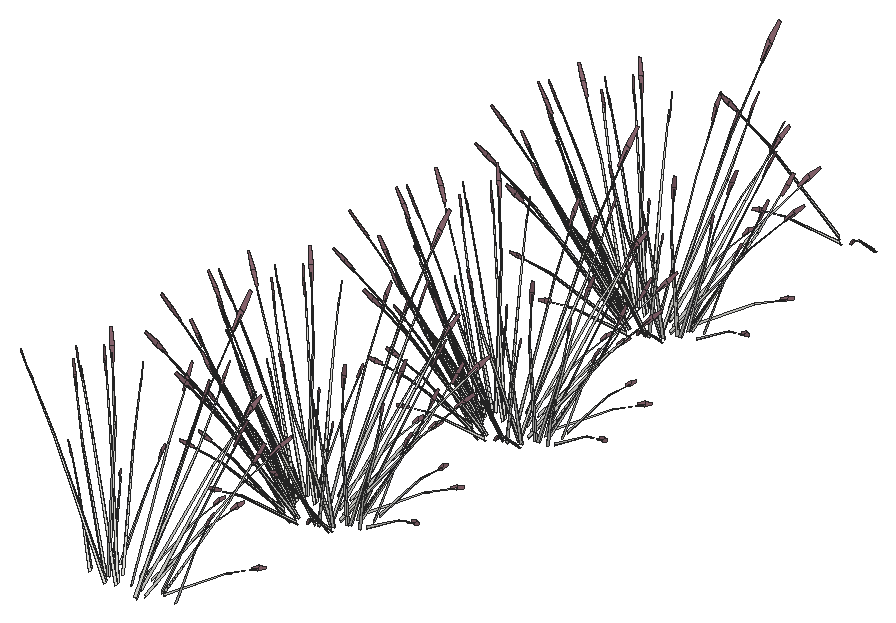
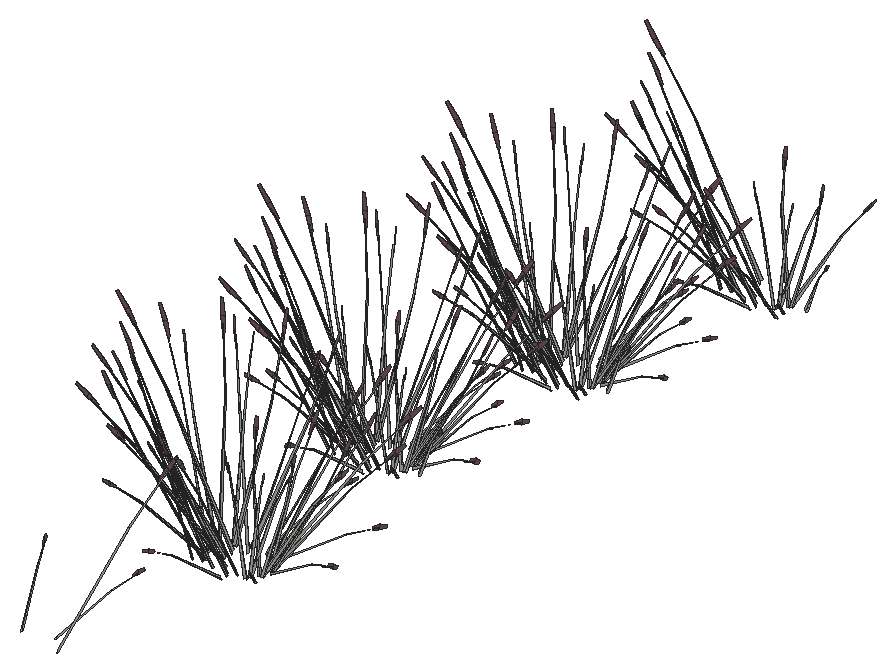
# SketchUp Ruby script. Lengths in inches.
U = 1.inch
M = Sketchup.active_model
def pt(a) = Geom::Point3d.new(a.map { |v| v * U })
def face(e, loops, mat)
  f = e.add_face(loops[0].map { |a| pt(a) })
  loops[1..].each { |l| e.add_face(l.map { |a| pt(a) }).erase! }
  f.material = f.back_material = mat if mat
  f
end
# faces: each face lists its corners as indices into pts; further lists are holes
def faces(e, pts, list, mat = nil) = list.each { |f| face(e, (f[0].is_a?(Array) ? f : [f]).map { |l| l.map { |i| pts[i] } }, mat) }
# xy, xz, yz: faces in a plane at the given z, y or x. An outline is a flat list of corners, or four numbers for a rectangle; further outlines are holes
def ring(l) = l.size == 4 ? [[l[0], l[1]], [l[2], l[1]], [l[2], l[3]], [l[0], l[3]]] : l.each_slice(2).to_a
def flat(e, list, mat, &to3) = list.each { |f| face(e, (f[0].is_a?(Array) ? f : [f]).map { |l| ring(l).map { |u, v| to3.(u, v) } }, mat) }
def xy(e, z, list, mat = nil) = flat(e, list, mat) { |x, y| [x, y, z] }
def xz(e, y, list, mat = nil) = flat(e, list, mat) { |x, z| [x, y, z] }
def yz(e, x, list, mat = nil) = flat(e, list, mat) { |y, z| [x, y, z] }
def lines(e, pts, list) = list.each { |a, b| e.add_line(pt(pts[a]), pt(pts[b])) }
# prism: a flat outline (further loops are holes) pulled along v
def prism(e, loops, v, mat = nil)
  f = face(e, loops, mat); d = Geom::Vector3d.new(v.map { |x| x * U })
  f.pushpull(f.normal.samedirection?(d) ? d.length : -d.length)
end
def box(e, o, s, mat = nil) = prism(e, [[o, [o[0] + s[0], o[1], o[2]], [o[0] + s[0], o[1] + s[1], o[2]], [o[0], o[1] + s[1], o[2]]]], [0, 0, s[2]], mat)
def at(x, y, z, deg = 0) = Geom::Transformation.translation(pt([x, y, z])) * Geom::Transformation.rotation(ORIGIN, Z_AXIS, deg.degrees)
def axes(o, x, y, z) = Geom::Transformation.new([*x, 0, *y, 0, *z, 0, *pt(o).to_a, 1])
def part(name) = M.definitions.add(name)
# library, detail: a bought-in or finely detailed component or shape, given as its bounding box
def library(name, o, s) = part(name).tap { |d| box(d.entities, o, s) }
def detail(e, o, s) = box(e.add_group.entities, o, s)
def put(e, d, t, mat = nil) = e.add_instance(d, t).tap { |i| i.material = mat if mat }
def group(e, t, mat = nil) = e.add_group.tap { |g| g.transformation = t; g.material = mat if mat }.entities
root = M.entities
M.materials.add("LightPink_Translucent").color = [144, 107, 117]
c1 = part("blade")
p = [[2.15,0.21,22],[0,0.17,0],[0.09,0.45,0],[2.18,0.31,22],[2.29,0.31,22],[0.38,0.45,0],
  [2.48,0.24,33],[2.49,0.24,33],[2.48,0.22,33]]
faces(c1.entities,p,[[0,1,2,3],[4,5,2,3],[6,3,4,7],[8,0,3,6]])
c2 = part("seeds")
p = [[0.3,-0.1,1.38],[-0.01,-0.03,1.59],[-0.01,-0.03,0.03],[0.14,-0.07,-0.07],[0.29,-0.03,3],[0.15,0.01,3.11]]
faces(c2.entities,p,[[0,1,2,3],[1,0,4,5]],"LightPink_Translucent")
c3 = part("blade with seeds")
put(c3.entities,c1,at(0,0,0))
put(c3.entities,c2,axes([2.4,0.25,30.99],[1.5799,-0.05474,1.17369],[-0.12525,1.92788,0.29478],[-0.07173,-0.02425,1.56792]))
put(root,c3,axes([41.28,395.99,45.93],[-0.23455,-0.87059,-0.03492],[1.10861,-0.20015,-0.15832],[0.23151,0.05519,0.52218]))
put(root,c3,axes([38.41,395.97,47.03],[0.06562,-1.05324,-0.1216],[1.2424,0.02879,-0.67495],[0.4785,0.07316,1.02557]))
put(root,c3,axes([39.49,395.34,46.72],[0.26289,-0.01751,1.74944],[0.72108,-0.8046,-0.27667],[0.46761,0.10621,0.14031]))
put(root,c3,axes([29.125,393.22,45.875],[0.42521,-0.21906,1.71376],[0.35798,1.01226,0.13857],[-0.66754,0.22878,0.73262]))
put(root,c3,axes([25.6,393.86,46.71],[0.1564,0.02778,1.77383],[0.48382,0.91506,-0.16761],[-0.32016,0.24017,0.31391]))
put(root,c3,axes([39.2,395.89,46.53],[0.69728,0.64842,-0.35414],[-0.79619,0.61382,0.4572],[0.40453,0.09339,0.87481]))
put(root,c3,axes([28.84,394.73,46.53],[-1.06674,0.14801,-0.35414],[-0.28168,-0.84611,0.4572],[-0.30569,0.22726,0.87481]))
put(root,c3,axes([36.7,394.23,45.875],[-0.45521,-0.17844,1.71376],[0.94204,-0.74856,0.13857],[0.58713,0.33769,0.73262]))
put(root,c3,axes([36.79,391.88,46.47],[-1.05895,-0.53811,1.38283],[1.11816,-0.83781,0.59665],[0.34166,0.5049,1.33663]))
put(root,c3,axes([29.15,394.15,47.03],[1.1336,0.57106,-0.1216],[-0.65308,0.827,-0.67495],[-0.32027,0.28747,1.02557]))
put(root,c3,axes([35.96,397.11,47.03],[0.73026,-0.88648,-0.1216],[1.05755,0.51071,-0.67495],[0.36761,0.25045,1.02557]))
put(root,c3,axes([30.68,393.9,45.875],[0.30609,-0.31822,1.71376],[0.77286,0.85893,0.13857],[-0.53009,0.39116,0.73262]))
put(root,c3,axes([35.01,397.85,46.71],[0.00363,-0.12539,1.77383],[1.0502,-0.55319,-0.16761],[0.36479,0.19745,0.31391]))
put(root,c3,axes([30.45,394.68,45.875],[0.22818,-0.35597,1.71376],[0.95725,0.73667,0.13857],[-0.43183,0.45914,0.73262]))
put(root,c3,axes([30.71,396.69,46.53],[-0.82919,0.54528,-0.35414],[-0.78493,-0.62262,0.4572],[-0.11943,0.31634,0.87481]))
put(root,c3,axes([27.86,396.53,46.72],[-0.03046,0.20495,1.74944],[0.86449,0.71297,-0.27667],[-0.22632,0.33716,0.14031]))
put(root,c3,axes([33.11,397.15,47.03],[1.19922,-0.48218,-0.1216],[0.58932,0.85579,-0.67495],[0.15822,0.36063,1.02557]))
put(root,c3,axes([34.82,395.27,45.875],[-0.28013,-0.33252,1.71376],[1.29445,-0.27994,0.13857],[0.29256,0.52202,0.73262]))
put(root,c3,axes([33.59,397.65,46.53],[-0.36946,0.79643,-0.35414],[-1.07787,-0.23229,0.4572],[0.09883,0.32066,0.87481]))
put(root,c3,axes([27.76,398.63,46.71],[0.13903,-0.06253,1.77383],[1.14912,0.41591,-0.16761],[-0.027,0.34629,0.31391]))
put(root,c3,axes([32.54,395.44,45.875],[-0.02999,-0.3975,1.71376],[1.30002,0.26369,0.13857],[-0.08041,0.56647,0.73262]))
put(root,c3,axes([32.83,399.06,46.72],[0.15534,0.16677,1.74944],[1.25362,0.06552,-0.27667],[0.12606,0.3678,0.14031]))
put(root,c3,axes([39.9,428.45,45.875],[0.28013,0.33252,1.71376],[-1.29445,0.27994,0.13857],[-0.29256,-0.52202,0.73262]))
put(root,c3,axes([42.04,426.25,46.72],[-0.18744,-0.14521,1.74944],[-1.25089,0.09206,-0.27667],[-0.19964,-0.34731,0.14031]))
put(root,c3,axes([47.66,428.03,46.72],[-0.01183,-0.20612,1.74944],[-0.99913,-0.59572,-0.27667],[0.15447,-0.36112,0.14031]))
put(root,c3,axes([43.46,427.98,46.53],[0.36946,-0.79643,-0.35414],[1.07787,0.23229,0.4572],[-0.09883,-0.32066,0.87481]))
put(root,c3,axes([44.28,429.04,45.875],[-0.22818,0.35597,1.71376],[-0.95725,-0.73667,0.13857],[0.43183,-0.45914,0.73262]))
put(root,c3,axes([47.39,427.29,46.71],[-0.12446,0.07911,1.77383],[-1.21937,-0.26689,-0.16761],[-0.04414,-0.34521,0.31391]))
put(root,c3,axes([40.76,425.77,46.71],[-0.02286,0.12414,1.77383],[-1.12758,0.45052,-0.16761],[-0.33182,-0.23029,0.31391]))
put(root,c3,axes([43.94,428.49,47.03],[-1.19922,0.48218,-0.1216],[-0.58932,-0.85579,-0.67495],[-0.15822,-0.36063,1.02557]))
put(root,c3,axes([46.43,429.57,47.03],[-1.34686,-0.05131,-0.1216],[0.03681,-0.97156,-0.67495],[0.09356,-0.37418,1.02557]))
put(root,c3,axes([46.34,428.95,46.53],[0.82919,-0.54528,-0.35414],[0.78493,0.62262,0.4572],[0.11943,-0.31634,0.87481]))
put(root,c3,axes([40.35,428.28,46.53],[-0.18927,-0.83419,-0.35414],[1.08199,-0.22027,0.4572],[-0.29062,-0.23905,0.87481]))
put(root,c3,axes([38.03,429.49,45.875],[0.45521,0.17844,1.71376],[-0.94204,0.74856,0.13857],[-0.58713,-0.33769,0.73262]))
put(root,c3,axes([37.9375,427.85,46.72],[-0.26368,-0.00731,1.74944],[-0.83946,0.73103,-0.27667],[-0.44791,-0.14937,0.14031]))
put(root,c3,axes([47.9,431.48,47.03],[-1.1336,-0.57106,-0.1216],[0.65308,-0.827,-0.67495],[0.32027,-0.28747,1.02557]))
put(root,c3,axes([50.69,431.24,46.71],[-0.16006,-0.00787,1.77383],[-0.66468,-0.8428,-0.16761],[0.26693,-0.27711,0.31391]))
put(root,c3,axes([48.22,430.91,46.53],[1.06674,-0.14801,-0.35414],[0.28168,0.84611,0.4572],[0.30569,-0.22726,0.87481]))
put(root,c3,axes([37.85,429.74,46.53],[-0.69728,-0.64842,-0.35414],[0.79619,-0.61382,0.4572],[-0.40453,-0.09339,0.87481]))
put(root,c3,axes([51.29,432.24,46.72],[0.17006,-0.15775,1.74944],[-0.21766,-0.96766,-0.27667],[0.42669,-0.18347,0.14031]))
put(root,c3,axes([36.92,428.47,46.71],[0.09085,0.10335,1.77383],[-0.43798,0.92907,-0.16761],[-0.44357,0.00672,0.31391]))
put(root,c3,axes([38.65,429.67,47.03],[-0.06562,1.05324,-0.1216],[-1.2424,-0.02879,-0.67495],[-0.4785,-0.07316,1.02557]))
put(root,c3,axes([47.94,433.71,47.03],[-0.6166,-0.93779,-0.1216],[1.09436,-0.46085,-0.67495],[0.46117,-0.12373,1.02557]))
put(root,c3,axes([37.07,431.12,45.875],[0.50831,-0.02346,1.71376],[-0.33721,1.01661,0.13857],[-0.72439,-0.06288,0.73262]))
put(root,c3,axes([48.59,433.34,46.53],[1.01846,0.28891,-0.35414],[-0.29705,0.84289,0.4572],[0.41005,-0.07729,0.87481]))
put(root,c3,axes([36.62,431.99,46.53],[-1.01846,-0.28891,-0.35414],[0.29705,-0.84289,0.4572],[-0.41005,0.07729,0.87481]))
put(root,c3,axes([45.8125,432.29,45.875],[-0.50831,0.02346,1.71376],[0.33721,-1.01661,0.13857],[0.72439,0.06288,0.73262]))
put(root,c3,axes([50.4,436.5,46.71],[-0.11081,-0.09067,1.77383],[0.2424,-0.97188,-0.16761],[0.43649,-0.06209,0.31391]))
put(root,c3,axes([35.98,432.55,46.72],[-0.20012,0.13446,1.74944],[0.01702,0.98243,-0.27667],[-0.45871,0.12776,0.14031]))
put(root,c3,axes([37.26,431.62,47.03],[0.6166,0.93779,-0.1216],[-1.09436,0.46085,-0.67495],[-0.46117,0.12373,1.02557]))
put(root,c3,axes([49.43,435.6875,45.93],[-0.23455,-0.87059,-0.03492],[1.10861,-0.20015,-0.15832],[0.23151,0.05519,0.52218]))
put(root,c3,axes([46.56,435.66,47.03],[0.06562,-1.05324,-0.1216],[1.2424,0.02879,-0.67495],[0.4785,0.07316,1.02557]))
put(root,c3,axes([47.64,435.03,46.72],[0.26289,-0.01751,1.74944],[0.72108,-0.8046,-0.27667],[0.46761,0.10621,0.14031]))
put(root,c3,axes([37.28,432.91,45.875],[0.42521,-0.21906,1.71376],[0.35798,1.01226,0.13857],[-0.66754,0.22878,0.73262]))
put(root,c3,axes([33.75,433.55,46.71],[0.1564,0.02778,1.77383],[0.48382,0.91506,-0.16761],[-0.32016,0.24017,0.31391]))
put(root,c3,axes([47.36,435.59,46.53],[0.69728,0.64842,-0.35414],[-0.79619,0.61382,0.4572],[0.40453,0.09339,0.87481]))
put(root,c3,axes([36.99,434.42,46.53],[-1.06674,0.14801,-0.35414],[-0.28168,-0.84611,0.4572],[-0.30569,0.22726,0.87481]))
put(root,c3,axes([44.85,433.92,45.875],[-0.45521,-0.17844,1.71376],[0.94204,-0.74856,0.13857],[0.58713,0.33769,0.73262]))
put(root,c3,axes([44.94,431.58,46.47],[-1.05895,-0.53811,1.38283],[1.11816,-0.83781,0.59665],[0.34166,0.5049,1.33663]))
put(root,c3,axes([37.31,433.85,47.03],[1.1336,0.57106,-0.1216],[-0.65308,0.827,-0.67495],[-0.32027,0.28747,1.02557]))
put(root,c3,axes([44.11,436.81,47.03],[0.73026,-0.88648,-0.1216],[1.05755,0.51071,-0.67495],[0.36761,0.25045,1.02557]))
put(root,c3,axes([38.83,433.59,45.875],[0.30609,-0.31822,1.71376],[0.77286,0.85893,0.13857],[-0.53009,0.39116,0.73262]))
put(root,c3,axes([43.16,437.54,46.71],[0.00363,-0.12539,1.77383],[1.0502,-0.55319,-0.16761],[0.36479,0.19745,0.31391]))
put(root,c3,axes([38.6,434.375,45.875],[0.22818,-0.35597,1.71376],[0.95725,0.73667,0.13857],[-0.43183,0.45914,0.73262]))
put(root,c3,axes([38.87,436.38,46.53],[-0.82919,0.54528,-0.35414],[-0.78493,-0.62262,0.4572],[-0.11943,0.31634,0.87481]))
put(root,c3,axes([36.01,436.22,46.72],[-0.03046,0.20495,1.74944],[0.86449,0.71297,-0.27667],[-0.22632,0.33716,0.14031]))
put(root,c3,axes([41.26,436.84,47.03],[1.19922,-0.48218,-0.1216],[0.58932,0.85579,-0.67495],[0.15822,0.36063,1.02557]))
put(root,c3,axes([42.98,434.96,45.875],[-0.28013,-0.33252,1.71376],[1.29445,-0.27994,0.13857],[0.29256,0.52202,0.73262]))
put(root,c3,axes([41.74,437.35,46.53],[-0.36946,0.79643,-0.35414],[-1.07787,-0.23229,0.4572],[0.09883,0.32066,0.87481]))
put(root,c3,axes([35.91,438.32,46.71],[0.13903,-0.06253,1.77383],[1.14912,0.41591,-0.16761],[-0.027,0.34629,0.31391]))
put(root,c3,axes([40.69,435.13,45.875],[-0.02999,-0.3975,1.71376],[1.30002,0.26369,0.13857],[-0.08041,0.56647,0.73262]))
put(root,c3,axes([40.98,438.76,46.72],[0.15534,0.16677,1.74944],[1.25362,0.06552,-0.27667],[0.12606,0.3678,0.14031]))
put(root,c3,axes([46.26,467.72,45.875],[0.28013,0.33252,1.71376],[-1.29445,0.27994,0.13857],[-0.29256,-0.52202,0.73262]))
put(root,c3,axes([48.39,465.51,46.72],[-0.18744,-0.14521,1.74944],[-1.25089,0.09206,-0.27667],[-0.19964,-0.34731,0.14031]))
put(root,c3,axes([54.01,467.29,46.72],[-0.01183,-0.20612,1.74944],[-0.99913,-0.59572,-0.27667],[0.15447,-0.36112,0.14031]))
put(root,c3,axes([49.82,467.25,46.53],[0.36946,-0.79643,-0.35414],[1.07787,0.23229,0.4572],[-0.09883,-0.32066,0.87481]))
put(root,c3,axes([50.63,468.3,45.875],[-0.22818,0.35597,1.71376],[-0.95725,-0.73667,0.13857],[0.43183,-0.45914,0.73262]))
put(root,c3,axes([47.11,465.04,46.71],[-0.02286,0.12414,1.77383],[-1.12758,0.45052,-0.16761],[-0.33182,-0.23029,0.31391]))
put(root,c3,axes([50.3,467.75,47.03],[-1.19922,0.48218,-0.1216],[-0.58932,-0.85579,-0.67495],[-0.15822,-0.36063,1.02557]))
put(root,c3,axes([52.79,468.84,47.03],[-1.34686,-0.05131,-0.1216],[0.03681,-0.97156,-0.67495],[0.09356,-0.37418,1.02557]))
put(root,c3,axes([52.69,468.21,46.53],[0.82919,-0.54528,-0.35414],[0.78493,0.62262,0.4572],[0.11943,-0.31634,0.87481]))
put(root,c3,axes([46.71,467.54,46.53],[-0.18927,-0.83419,-0.35414],[1.08199,-0.22027,0.4572],[-0.29062,-0.23905,0.87481]))
put(root,c3,axes([44.38,468.75,45.875],[0.45521,0.17844,1.71376],[-0.94204,0.74856,0.13857],[-0.58713,-0.33769,0.73262]))
put(root,c3,axes([44.29,467.11,46.72],[-0.26368,-0.00731,1.74944],[-0.83946,0.73103,-0.27667],[-0.44791,-0.14937,0.14031]))
put(root,c3,axes([54.25,470.75,47.03],[-1.1336,-0.57106,-0.1216],[0.65308,-0.827,-0.67495],[0.32027,-0.28747,1.02557]))
put(root,c3,axes([57.05,470.5,46.71],[-0.16006,-0.00787,1.77383],[-0.66468,-0.8428,-0.16761],[0.26693,-0.27711,0.31391]))
put(root,c3,axes([54.57,470.17,46.53],[1.06674,-0.14801,-0.35414],[0.28168,0.84611,0.4572],[0.30569,-0.22726,0.87481]))
put(root,c3,axes([44.2,469.01,46.53],[-0.69728,-0.64842,-0.35414],[0.79619,-0.61382,0.4572],[-0.40453,-0.09339,0.87481]))
put(root,c3,axes([57.65,471.51,46.72],[0.17006,-0.15775,1.74944],[-0.21766,-0.96766,-0.27667],[0.42669,-0.18347,0.14031]))
put(root,c3,axes([43.28,467.73,46.71],[0.09085,0.10335,1.77383],[-0.43798,0.92907,-0.16761],[-0.44357,0.00672,0.31391]))
put(root,c3,axes([45,468.93,47.03],[-0.06562,1.05324,-0.1216],[-1.2424,-0.02879,-0.67495],[-0.4785,-0.07316,1.02557]))
put(root,c3,axes([54.3,472.98,47.03],[-0.6166,-0.93779,-0.1216],[1.09436,-0.46085,-0.67495],[0.46117,-0.12373,1.02557]))
put(root,c3,axes([43.42,470.39,45.875],[0.50831,-0.02346,1.71376],[-0.33721,1.01661,0.13857],[-0.72439,-0.06288,0.73262]))
put(root,c3,axes([54.94,472.6,46.53],[1.01846,0.28891,-0.35414],[-0.29705,0.84289,0.4572],[0.41005,-0.07729,0.87481]))
put(root,c3,axes([42.97,471.26,46.53],[-1.01846,-0.28891,-0.35414],[0.29705,-0.84289,0.4572],[-0.41005,0.07729,0.87481]))
put(root,c3,axes([52.17,471.56,45.875],[-0.50831,0.02346,1.71376],[0.33721,-1.01661,0.13857],[0.72439,0.06288,0.73262]))
put(root,c3,axes([56.75,475.76,46.71],[-0.11081,-0.09067,1.77383],[0.2424,-0.97188,-0.16761],[0.43649,-0.06209,0.31391]))
put(root,c3,axes([42.33,471.82,46.72],[-0.20012,0.13446,1.74944],[0.01702,0.98243,-0.27667],[-0.45871,0.12776,0.14031]))
put(root,c3,axes([43.62,470.88,47.03],[0.6166,0.93779,-0.1216],[-1.09436,0.46085,-0.67495],[-0.46117,0.12373,1.02557]))
put(root,c3,axes([55.79,474.95,45.93],[-0.23455,-0.87059,-0.03492],[1.10861,-0.20015,-0.15832],[0.23151,0.05519,0.52218]))
put(root,c3,axes([52.92,474.93,47.03],[0.06562,-1.05324,-0.1216],[1.2424,0.02879,-0.67495],[0.4785,0.07316,1.02557]))
put(root,c3,axes([54,474.29,46.72],[0.26289,-0.01751,1.74944],[0.72108,-0.8046,-0.27667],[0.46761,0.10621,0.14031]))
put(root,c3,axes([43.63,472.17,45.875],[0.42521,-0.21906,1.71376],[0.35798,1.01226,0.13857],[-0.66754,0.22878,0.73262]))
put(root,c3,axes([40.11,472.8125,46.71],[0.1564,0.02778,1.77383],[0.48382,0.91506,-0.16761],[-0.32016,0.24017,0.31391]))
put(root,c3,axes([53.71,474.85,46.53],[0.69728,0.64842,-0.35414],[-0.79619,0.61382,0.4572],[0.40453,0.09339,0.87481]))
put(root,c3,axes([43.35,473.6875,46.53],[-1.06674,0.14801,-0.35414],[-0.28168,-0.84611,0.4572],[-0.30569,0.22726,0.87481]))
put(root,c3,axes([51.21,473.19,45.875],[-0.45521,-0.17844,1.71376],[0.94204,-0.74856,0.13857],[0.58713,0.33769,0.73262]))
put(root,c3,axes([51.3,470.84,46.47],[-1.05895,-0.53811,1.38283],[1.11816,-0.83781,0.59665],[0.34166,0.5049,1.33663]))
put(root,c3,axes([43.66,473.11,47.03],[1.1336,0.57106,-0.1216],[-0.65308,0.827,-0.67495],[-0.32027,0.28747,1.02557]))
put(root,c3,axes([50.47,476.07,47.03],[0.73026,-0.88648,-0.1216],[1.05755,0.51071,-0.67495],[0.36761,0.25045,1.02557]))
put(root,c3,axes([45.1875,472.86,45.875],[0.30609,-0.31822,1.71376],[0.77286,0.85893,0.13857],[-0.53009,0.39116,0.73262]))
put(root,c3,axes([49.51,476.81,46.71],[0.00363,-0.12539,1.77383],[1.0502,-0.55319,-0.16761],[0.36479,0.19745,0.31391]))
put(root,c3,axes([44.96,473.64,45.875],[0.22818,-0.35597,1.71376],[0.95725,0.73667,0.13857],[-0.43183,0.45914,0.73262]))
put(root,c3,axes([45.22,475.65,46.53],[-0.82919,0.54528,-0.35414],[-0.78493,-0.62262,0.4572],[-0.11943,0.31634,0.87481]))
put(root,c3,axes([42.36,475.49,46.72],[-0.03046,0.20495,1.74944],[0.86449,0.71297,-0.27667],[-0.22632,0.33716,0.14031]))
put(root,c3,axes([47.62,476.11,47.03],[1.19922,-0.48218,-0.1216],[0.58932,0.85579,-0.67495],[0.15822,0.36063,1.02557]))
put(root,c3,axes([49.33,474.23,45.875],[-0.28013,-0.33252,1.71376],[1.29445,-0.27994,0.13857],[0.29256,0.52202,0.73262]))
put(root,c3,axes([48.1,476.61,46.53],[-0.36946,0.79643,-0.35414],[-1.07787,-0.23229,0.4572],[0.09883,0.32066,0.87481]))
put(root,c3,axes([47.05,474.39,45.875],[-0.02999,-0.3975,1.71376],[1.30002,0.26369,0.13857],[-0.08041,0.56647,0.73262]))
put(root,c3,axes([47.34,478.02,46.72],[0.15534,0.16677,1.74944],[1.25362,0.06552,-0.27667],[0.12606,0.3678,0.14031]))
put(root,c3,axes([42.64,507.97,45.875],[0.28013,0.33252,1.71376],[-1.29445,0.27994,0.13857],[-0.29256,-0.52202,0.73262]))
put(root,c3,axes([44.78,505.77,46.72],[-0.18744,-0.14521,1.74944],[-1.25089,0.09206,-0.27667],[-0.19964,-0.34731,0.14031]))
put(root,c3,axes([50.4,507.55,46.72],[-0.01183,-0.20612,1.74944],[-0.99913,-0.59572,-0.27667],[0.15447,-0.36112,0.14031]))
put(root,c3,axes([46.2,507.51,46.53],[0.36946,-0.79643,-0.35414],[1.07787,0.23229,0.4572],[-0.09883,-0.32066,0.87481]))
put(root,c3,axes([47.02,508.5625,45.875],[-0.22818,0.35597,1.71376],[-0.95725,-0.73667,0.13857],[0.43183,-0.45914,0.73262]))
put(root,c3,axes([46.68,508.01,47.03],[-1.19922,0.48218,-0.1216],[-0.58932,-0.85579,-0.67495],[-0.15822,-0.36063,1.02557]))
put(root,c3,axes([49.17,509.09,47.03],[-1.34686,-0.05131,-0.1216],[0.03681,-0.97156,-0.67495],[0.09356,-0.37418,1.02557]))
put(root,c3,axes([49.08,508.47,46.53],[0.82919,-0.54528,-0.35414],[0.78493,0.62262,0.4572],[0.11943,-0.31634,0.87481]))
put(root,c3,axes([43.09,507.8,46.53],[-0.18927,-0.83419,-0.35414],[1.08199,-0.22027,0.4572],[-0.29062,-0.23905,0.87481]))
put(root,c3,axes([40.77,509.01,45.875],[0.45521,0.17844,1.71376],[-0.94204,0.74856,0.13857],[-0.58713,-0.33769,0.73262]))
put(root,c3,axes([40.68,507.37,46.72],[-0.26368,-0.00731,1.74944],[-0.83946,0.73103,-0.27667],[-0.44791,-0.14937,0.14031]))
put(root,c3,axes([50.64,511.01,47.03],[-1.1336,-0.57106,-0.1216],[0.65308,-0.827,-0.67495],[0.32027,-0.28747,1.02557]))
put(root,c3,axes([50.96,510.43,46.53],[1.06674,-0.14801,-0.35414],[0.28168,0.84611,0.4572],[0.30569,-0.22726,0.87481]))
put(root,c3,axes([40.59,509.27,46.53],[-0.69728,-0.64842,-0.35414],[0.79619,-0.61382,0.4572],[-0.40453,-0.09339,0.87481]))
put(root,c3,axes([54.03,511.77,46.72],[0.17006,-0.15775,1.74944],[-0.21766,-0.96766,-0.27667],[0.42669,-0.18347,0.14031]))
put(root,c3,axes([41.39,509.19,47.03],[-0.06562,1.05324,-0.1216],[-1.2424,-0.02879,-0.67495],[-0.4785,-0.07316,1.02557]))
put(root,c3,axes([50.69,513.24,47.03],[-0.6166,-0.93779,-0.1216],[1.09436,-0.46085,-0.67495],[0.46117,-0.12373,1.02557]))
put(root,c3,axes([39.81,510.64,45.875],[0.50831,-0.02346,1.71376],[-0.33721,1.01661,0.13857],[-0.72439,-0.06288,0.73262]))
put(root,c3,axes([51.33,512.86,46.53],[1.01846,0.28891,-0.35414],[-0.29705,0.84289,0.4572],[0.41005,-0.07729,0.87481]))
put(root,c3,axes([39.36,511.52,46.53],[-1.01846,-0.28891,-0.35414],[0.29705,-0.84289,0.4572],[-0.41005,0.07729,0.87481]))
put(root,c3,axes([48.55,511.82,45.875],[-0.50831,0.02346,1.71376],[0.33721,-1.01661,0.13857],[0.72439,0.06288,0.73262]))
put(root,c3,axes([38.72,512.08,46.72],[-0.20012,0.13446,1.74944],[0.01702,0.98243,-0.27667],[-0.45871,0.12776,0.14031]))
put(root,c3,axes([40,511.14,47.03],[0.6166,0.93779,-0.1216],[-1.09436,0.46085,-0.67495],[-0.46117,0.12373,1.02557]))
put(root,c3,axes([52.17,515.21,45.93],[-0.23455,-0.87059,-0.03492],[1.10861,-0.20015,-0.15832],[0.23151,0.05519,0.52218]))
put(root,c3,axes([49.3,515.18,47.03],[0.06562,-1.05324,-0.1216],[1.2424,0.02879,-0.67495],[0.4785,0.07316,1.02557]))
put(root,c3,axes([50.38,514.55,46.72],[0.26289,-0.01751,1.74944],[0.72108,-0.8046,-0.27667],[0.46761,0.10621,0.14031]))
put(root,c3,axes([40.02,512.43,45.875],[0.42521,-0.21906,1.71376],[0.35798,1.01226,0.13857],[-0.66754,0.22878,0.73262]))
put(root,c3,axes([50.1,515.11,46.53],[0.69728,0.64842,-0.35414],[-0.79619,0.61382,0.4572],[0.40453,0.09339,0.87481]))
put(root,c3,axes([39.73,513.95,46.53],[-1.06674,0.14801,-0.35414],[-0.28168,-0.84611,0.4572],[-0.30569,0.22726,0.87481]))
put(root,c3,axes([47.59,513.45,45.875],[-0.45521,-0.17844,1.71376],[0.94204,-0.74856,0.13857],[0.58713,0.33769,0.73262]))
put(root,c3,axes([47.68,511.1,46.47],[-1.05895,-0.53811,1.38283],[1.11816,-0.83781,0.59665],[0.34166,0.5049,1.33663]))
put(root,c3,axes([40.05,513.37,47.03],[1.1336,0.57106,-0.1216],[-0.65308,0.827,-0.67495],[-0.32027,0.28747,1.02557]))
put(root,c3,axes([46.85,516.33,47.03],[0.73026,-0.88648,-0.1216],[1.05755,0.51071,-0.67495],[0.36761,0.25045,1.02557]))
put(root,c3,axes([41.57,513.11,45.875],[0.30609,-0.31822,1.71376],[0.77286,0.85893,0.13857],[-0.53009,0.39116,0.73262]))
put(root,c3,axes([41.34,513.9,45.875],[0.22818,-0.35597,1.71376],[0.95725,0.73667,0.13857],[-0.43183,0.45914,0.73262]))
put(root,c3,axes([41.61,515.91,46.53],[-0.82919,0.54528,-0.35414],[-0.78493,-0.62262,0.4572],[-0.11943,0.31634,0.87481]))
put(root,c3,axes([38.75,515.75,46.72],[-0.03046,0.20495,1.74944],[0.86449,0.71297,-0.27667],[-0.22632,0.33716,0.14031]))
put(root,c3,axes([44,516.37,47.03],[1.19922,-0.48218,-0.1216],[0.58932,0.85579,-0.67495],[0.15822,0.36063,1.02557]))
put(root,c3,axes([45.72,514.49,45.875],[-0.28013,-0.33252,1.71376],[1.29445,-0.27994,0.13857],[0.29256,0.52202,0.73262]))
put(root,c3,axes([44.49,516.87,46.53],[-0.36946,0.79643,-0.35414],[-1.07787,-0.23229,0.4572],[0.09883,0.32066,0.87481]))
put(root,c3,axes([43.43,514.65,45.875],[-0.02999,-0.3975,1.71376],[1.30002,0.26369,0.13857],[-0.08041,0.56647,0.73262]))
put(root,c3,axes([43.72,518.28,46.72],[0.15534,0.16677,1.74944],[1.25362,0.06552,-0.27667],[0.12606,0.3678,0.14031]))
put(root,c3,axes([50.61,551.65,45.875],[0.28013,0.33252,1.71376],[-1.29445,0.27994,0.13857],[-0.29256,-0.52202,0.73262]))
put(root,c3,axes([52.75,549.45,46.72],[-0.18744,-0.14521,1.74944],[-1.25089,0.09206,-0.27667],[-0.19964,-0.34731,0.14031]))
put(root,c3,axes([58.37,551.23,46.72],[-0.01183,-0.20612,1.74944],[-0.99913,-0.59572,-0.27667],[0.15447,-0.36112,0.14031]))
